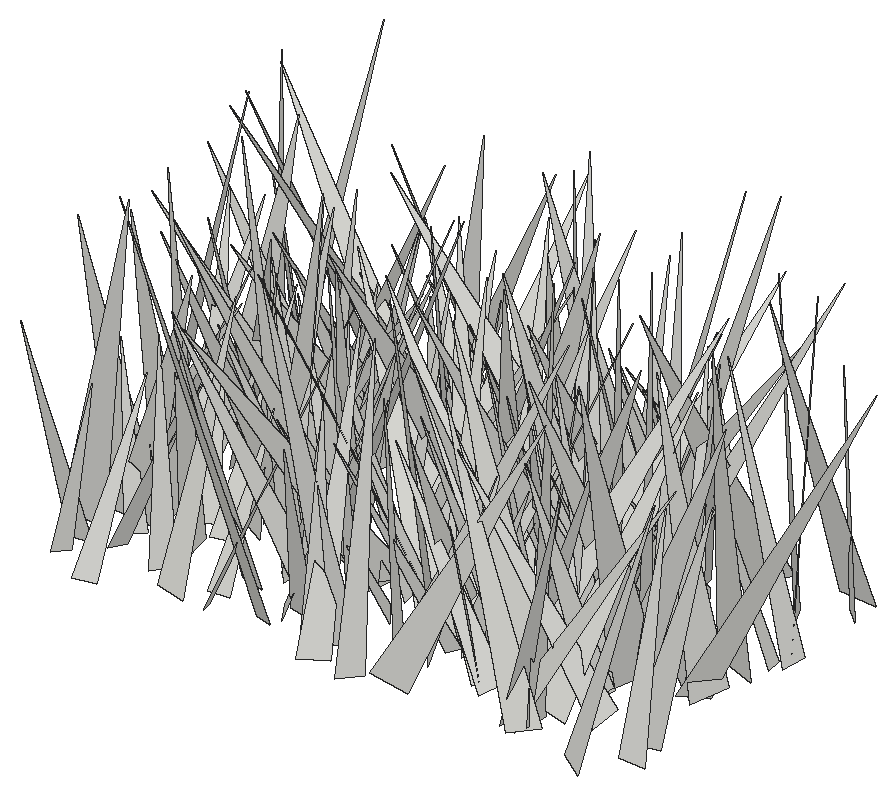
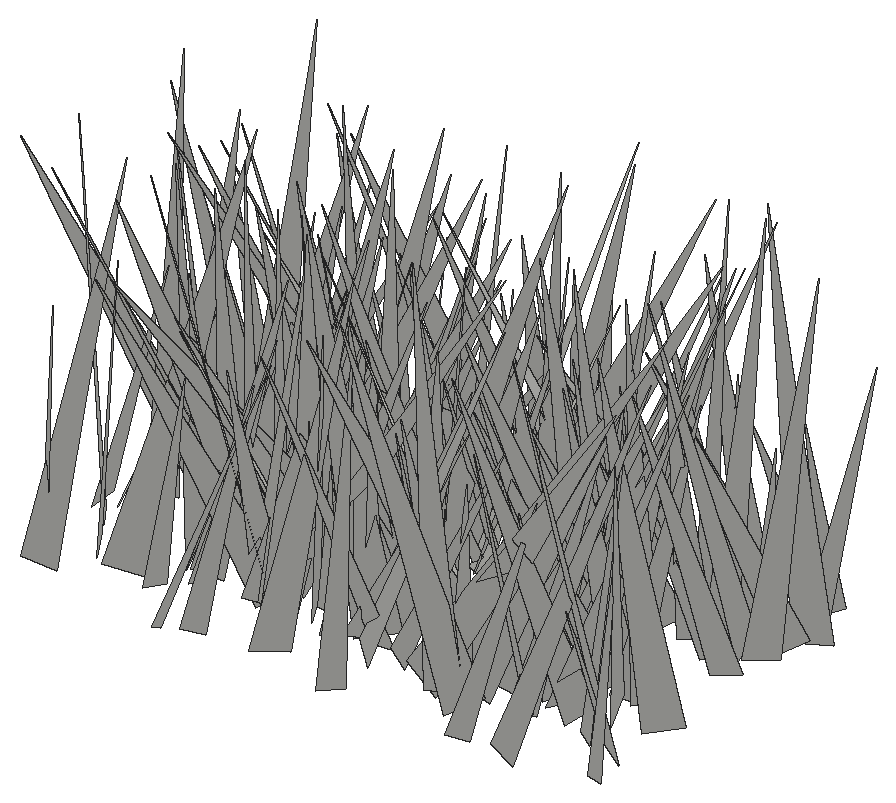
# SketchUp Ruby script. Lengths in inches.
U = 1.inch
M = Sketchup.active_model
def pt(a) = Geom::Point3d.new(a.map { |v| v * U })
def face(e, loops, mat)
  f = e.add_face(loops[0].map { |a| pt(a) })
  loops[1..].each { |l| e.add_face(l.map { |a| pt(a) }).erase! }
  f.material = f.back_material = mat if mat
  f
end
# faces: each face lists its corners as indices into pts; further lists are holes
def faces(e, pts, list, mat = nil) = list.each { |f| face(e, (f[0].is_a?(Array) ? f : [f]).map { |l| l.map { |i| pts[i] } }, mat) }
# xy, xz, yz: faces in a plane at the given z, y or x. An outline is a flat list of corners, or four numbers for a rectangle; further outlines are holes
def ring(l) = l.size == 4 ? [[l[0], l[1]], [l[2], l[1]], [l[2], l[3]], [l[0], l[3]]] : l.each_slice(2).to_a
def flat(e, list, mat, &to3) = list.each { |f| face(e, (f[0].is_a?(Array) ? f : [f]).map { |l| ring(l).map { |u, v| to3.(u, v) } }, mat) }
def xy(e, z, list, mat = nil) = flat(e, list, mat) { |x, y| [x, y, z] }
def xz(e, y, list, mat = nil) = flat(e, list, mat) { |x, z| [x, y, z] }
def yz(e, x, list, mat = nil) = flat(e, list, mat) { |y, z| [x, y, z] }
def lines(e, pts, list) = list.each { |a, b| e.add_line(pt(pts[a]), pt(pts[b])) }
# prism: a flat outline (further loops are holes) pulled along v
def prism(e, loops, v, mat = nil)
  f = face(e, loops, mat); d = Geom::Vector3d.new(v.map { |x| x * U })
  f.pushpull(f.normal.samedirection?(d) ? d.length : -d.length)
end
def box(e, o, s, mat = nil) = prism(e, [[o, [o[0] + s[0], o[1], o[2]], [o[0] + s[0], o[1] + s[1], o[2]], [o[0], o[1] + s[1], o[2]]]], [0, 0, s[2]], mat)
def at(x, y, z, deg = 0) = Geom::Transformation.translation(pt([x, y, z])) * Geom::Transformation.rotation(ORIGIN, Z_AXIS, deg.degrees)
def axes(o, x, y, z) = Geom::Transformation.new([*x, 0, *y, 0, *z, 0, *pt(o).to_a, 1])
def part(name) = M.definitions.add(name)
# library, detail: a bought-in or finely detailed component or shape, given as its bounding box
def library(name, o, s) = part(name).tap { |d| box(d.entities, o, s) }
def detail(e, o, s) = box(e.add_group.entities, o, s)
def put(e, d, t, mat = nil) = e.add_instance(d, t).tap { |i| i.material = mat if mat }
def group(e, t, mat = nil) = e.add_group.tap { |g| g.transformation = t; g.material = mat if mat }.entities
root = M.entities
c1 = part("fur_instance\#9")
p = [[0.8125,0,1.79],[0.67,-0.02,1.48],[0,-0.11,0],[0,0.11,0]]
faces(c1.entities,p,[[0,1,2,3]])
put(root,c1,axes([545.91,126.66,-21.86],[5.53978,-0.90724,0.62547],[-0.85463,-5.56113,-0.49688],[-0.69563,-0.39269,5.59154]))
put(root,c1,axes([535.66,127.86,-21.86],[0.2783,-5.0487,0.14304],[-4.93686,-0.24166,1.07529],[1.0664,0.19877,4.94071]))
put(root,c1,axes([526.28,127.23,-21.86],[-0.19346,-4.85951,0.89963],[-4.92735,0.1202,-0.41034],[-0.38132,0.91231,4.84602]))
put(root,c1,axes([549.55,125.37,-21.86],[2.91311,4.64162,1.0633],[4.76072,-2.81168,-0.76908],[0.10392,-1.30816,5.4258]))
put(root,c1,axes([526.26,126.17,-21.86],[3.08181,-1.73974,0.98019],[-1.88437,-3.1302,0.36886],[-0.66077,0.81254,3.51969]))
put(root,c1,axes([546.97,125.95,-21.66],[-2.40654,5.51072,1.54274],[5.60544,1.9331,1.83892],[-1.15197,-2.10585,5.72519]))
put(root,c1,axes([528.22,124.99,-21.86],[-2.24412,3.20659,0.81725],[3.00578,2.38826,-1.11699],[1.38398,0.01256,3.75108]))
put(root,c1,axes([538.11,126.98,-21.86],[-0.62718,-6.98929,2.39617],[-7.29856,0.2117,-1.29283],[-1.15016,2.46782,6.89725]))
put(root,c1,axes([540.98,125.93,-21.86],[3.61026,-5.57217,1.81458],[-5.57053,-2.60139,3.09478],[1.81959,3.09184,5.87413]))
put(root,c1,axes([537.15,126.65,-21.86],[-2.61332,3.50076,2.27341],[3.90248,3.00092,-0.13507],[1.48133,-1.72983,4.36652]))
put(root,c1,axes([534.79,126.73,-21.86],[-5.1387,-6.17044,1.38685],[-6.22365,4.61615,-2.52214],[-1.12419,2.64967,7.62361]))
put(root,c1,axes([542.95,128.45,-21.86],[-2.708,-3.38854,1.07596],[-2.8715,2.88211,1.84961],[2.09627,-0.42942,3.92357]))
put(root,c1,axes([539.9,125.13,-21.66],[-5.67085,1.89535,1.35099],[1.57668,5.74544,-1.44226],[1.71219,0.98676,5.80265]))
put(root,c1,axes([532.86,128.52,-21.86],[-1.81224,-5.34948,0.90018],[-5.42401,1.80193,-0.21131],[0.08596,0.92064,5.64415]))
put(root,c1,axes([525.4,128.48,-21.86],[1.45469,-7.67033,1.86376],[-7.74266,-1.0178,1.85445],[1.53584,2.13396,7.5836]))
put(root,c1,axes([531.04,126.22,-21.86],[0.94432,5.62245,1.27282],[5.76049,-0.87093,-0.42662],[0.22085,-1.32412,5.68522]))
put(root,c1,axes([548.68,128.33,-21.66],[-5.67147,0.82087,0.04901],[0.80443,5.46726,1.5178],[-0.17066,-1.50898,5.5259]))
put(root,c1,axes([545.83,126.66,-21.86],[3.84668,4.92623,0.09388],[4.62666,-3.57049,-2.21792],[1.69428,-1.43435,5.84342]))
put(root,c1,axes([551.09,126.8,-21.86],[-0.27729,4.76979,1.49646],[4.98187,0.38774,-0.31274],[0.41383,-1.47171,4.7676]))
put(root,c1,axes([534.89,129.3125,-21.86],[-6.28485,-0.79991,0.77187],[-0.56549,6.11624,1.73401],[0.95701,-1.63912,6.09364]))
put(root,c1,axes([536.53,131.54,-21.86],[4.16443,-6.48584,0.7003],[-5.50995,-3.94185,-3.74183],[-3.49241,-1.51483,6.7385]))
put(root,c1,axes([529.8,127.38,-21.86],[3.42061,-2.16163,2.16053],[-2.46149,-3.8706,0.02453],[-1.81151,1.17767,4.04631]))
put(root,c1,axes([544.05,127.85,-21.86],[-4.37284,2.10544,0.41102],[2.13916,4.20984,1.19366],[-0.16073,-1.25217,4.70423]))
put(root,c1,axes([541.25,130.33,-21.66],[5.27025,-2.47106,0.85487],[-2.00329,-5.05203,-2.25305],[-1.68041,-1.72721,5.36707]))
put(root,c1,axes([537.88,125.61,-21.86],[-5.09281,3.29268,0.78292],[3.01884,5.05892,-1.63872],[1.53013,0.9783,5.83893]))
put(root,c1,axes([537.95,129.79,-21.86],[-3.80651,-3.12707,0.03174],[-3.06593,3.74155,0.93273],[0.61617,-0.70095,4.83716]))
put(root,c1,axes([540.84,128.29,-21.86],[3.81482,2.67004,0.71919],[2.75746,-3.58156,-1.32965],[0.20681,-1.49748,4.4625]))
put(root,c1,axes([532.44,127.17,-21.86],[-1.29453,3.3269,0.92168],[3.25121,1.50588,-0.8692],[1.16077,-0.50757,3.46245]))
put(root,c1,axes([550.69,127.96,-21.86],[3.34726,-4.07819,1.53745],[-4.35777,-3.09938,1.26621],[0.07255,1.99042,5.12177]))
put(root,c1,axes([547.47,129.55,-21.66],[-4.78026,1.17069,2.19317],[1.89155,4.79719,1.56216],[1.61324,-2.15588,4.66702]))
put(root,c1,axes([526.73,129.53,-21.86],[2.49015,-6.48815,0.76577],[-6.33726,-2.19962,1.97082],[1.58797,1.39602,6.66429]))
put(root,c1,axes([545.3,128.73,-21.66],[3.76435,-5.16952,3.38659],[-5.24976,-4.76711,-1.44149],[-3.26082,1.70703,6.23028]))
put(root,c1,axes([540.42,127.59,-21.86],[4.07945,6.65627,1.20942],[6.56454,-3.55321,-2.58689],[1.63565,-2.3408,7.36585]))
put(root,c1,axes([539.65,128.14,-21.86],[-4.30965,-1.39305,1.63599],[-1.58025,4.5392,-0.29767],[1.45598,0.80324,4.51941]))
put(root,c1,axes([527.98,130.34,-21.66],[6.98441,-2.34407,2.00985],[-1.86712,-7.16517,-1.86827],[-2.45928,-1.21733,7.12645]))
put(root,c1,axes([529.87,128.97,-21.86],[-7.27615,-1.41209,3.18772],[-1.2687,7.94356,0.62294],[3.24745,-0.06052,7.38568]))
put(root,c1,axes([541.52,128.89,-21.66],[-1.12844,-4.06047,0.83548],[-3.60524,0.5338,-2.27512],[-2.04639,1.29864,3.54749]))
put(root,c1,axes([547.48,131.46,-21.86],[6.81384,-4.6319,0.82302],[-4.34734,-6.75311,-2.01405],[-1.7979,-1.22528,7.98915]))
put(root,c1,axes([546.91,126.72,-21.66],[-7.37531,-1.40171,2.74866],[-2.16749,7.42249,-2.03071],[2.19589,2.61858,7.22747]))
put(root,c1,axes([543.5,128.16,-21.86],[-3.62089,2.64212,0.01483],[2.58278,3.53416,0.96476],[-0.55698,-0.78788,4.37731]))
put(root,c1,axes([537.35,132.18,-21.66],[-4.65731,-6.85842,0.0184],[-6.74044,4.58127,1.51895],[1.26677,-0.83835,8.14992]))
put(root,c1,axes([525.89,130.72,-21.66],[5.91516,-3.3432,1.65321],[-2.9566,-6.09276,-1.74243],[-2.27346,-0.77492,6.56735]))
put(root,c1,axes([543.75,129.52,-21.86],[-0.61117,-4.98438,1.28841],[-4.9544,0.21679,-1.51148],[-1.3993,1.40945,4.78884]))
put(root,c1,axes([539.55,130.21,-21.86],[-4.05006,-5.82532,2.03849],[-5.82326,4.4146,1.04584],[2.04438,1.03428,7.01738]))
put(root,c1,axes([527.52,128.74,-21.86],[-2.21806,2.84038,1.31516],[3.07662,2.27502,0.2754],[0.57601,-1.21396,3.59328]))
put(root,c1,axes([537.99,127.83,-21.66],[-6.10428,-1.79449,1.71008],[-2.20054,6.01533,-1.54278],[1.14113,2.0006,6.1727]))
put(root,c1,axes([527.43,127.86,-21.86],[4.11341,0.99659,0.14821],[0.94897,-4.04143,0.83763],[-0.33855,0.78037,4.1487]))
put(root,c1,axes([541.73,129.39,-21.66],[0.78956,-4.05986,1.16414],[-3.93825,-0.27989,1.69498],[1.52574,1.37851,3.77266]))
put(root,c1,axes([544.34,129.38,-21.86],[5.3173,-1.56529,0.48292],[-1.59322,-5.32309,0.28875],[-0.38078,0.41424,5.53538]))
put(root,c1,axes([527.8,127.38,-21.66],[5.78446,0.51407,0.77192],[0.25637,-5.57234,1.78981],[-0.89129,1.73346,5.52457]))
put(root,c1,axes([532.67,126.25,-21.86],[5.39727,3.08007,0.18691],[2.81936,-5.07536,2.22356],[-1.25418,1.84558,5.80286]))
put(root,c1,axes([546.83,127.5,-21.66],[0.07577,6.70614,0.84141],[6.48392,0.16538,-1.90197],[1.90764,-0.82847,6.43122]))
put(root,c1,axes([541.76,130.47,-21.86],[0.99148,-3.49866,0.36174],[-3.47594,-0.91715,0.65665],[0.53788,0.52224,3.57665]))
put(root,c1,axes([535.07,131.43,-21.86],[-0.95701,-7.3765,1.52863],[-7.35851,1.24531,1.40248],[1.61303,1.30453,7.30491]))
put(root,c1,axes([525.54,129.35,-21.66],[4.06898,-3.86093,0.67624],[-3.71406,-3.48612,2.44405],[1.25293,2.20473,5.04877]))
put(root,c1,axes([536.17,131.25,-21.86],[-0.88156,-7.55851,1.51866],[-6.98391,0.13553,-3.37952],[-3.26533,1.75074,6.81814]))
put(root,c1,axes([545.95,128.66,-21.86],[-5.8174,-1.77979,0.63377],[-1.88895,5.44209,-2.05595],[-0.03436,2.15114,5.72563]))
put(root,c1,axes([546.76,133.03,-21.86],[4.80853,-5.64104,1.01196],[-5.19564,-4.8483,-2.3381],[-2.41883,-0.80002,7.03396]))
put(root,c1,axes([535.25,127.27,-21.66],[6.47525,4.61232,0.40047],[4.47579,-6.41261,1.48613],[-1.18373,0.98374,7.80985]))
put(root,c1,axes([531.86,132.4,-21.86],[0.11863,-7.1905,0.64579],[-7.08435,-0.24031,-1.37429],[-1.39009,0.61104,7.05894]))
put(root,c1,axes([547.37,129.81,-21.86],[-5.94659,0.26274,1.16381],[0.1992,6.05181,-0.34844],[1.17635,0.30341,5.94219]))
put(root,c1,axes([541.85,132.21,-21.86],[-5.8383,-2.13052,1.19785],[-1.77007,5.82456,1.73238],[1.68547,-1.263,5.96857]))
put(root,c1,axes([542.11,129.29,-21.86],[-2.40389,3.30252,0.08348],[3.28439,2.37806,0.4999],[-0.35549,-0.36124,4.05406]))
put(root,c1,axes([547.38,131.37,-21.66],[1.03631,-6.95808,1.71035],[-6.57848,-0.23906,3.0134],[2.83968,1.98547,6.35675]))
put(root,c1,axes([545.26,130.74,-21.86],[3.00481,-2.76961,0.12717],[-2.71494,-2.90128,0.96303],[0.56213,0.79222,3.97142]))
put(root,c1,axes([539.18,130.71,-21.86],[-0.30638,-3.92044,1.36874],[-3.76361,-0.31774,-1.75256],[-1.75458,1.36615,3.52026]))
put(root,c1,axes([544.57,129.3,-21.86],[3.86177,3.77021,1.4507],[3.73701,-4.09632,0.69796],[-1.5342,-0.48777,5.35169]))
put(root,c1,axes([543.65,130.46,-21.86],[-6.06762,4.08752,0.30456],[4.00596,5.79855,1.98636],[-0.86766,-1.81261,7.04117]))
put(root,c1,axes([533.8125,131.25,-21.66],[-0.35504,-4.51922,1.36303],[-4.31721,-0.2418,-1.92625],[-1.90863,1.3876,4.10353]))
put(root,c1,axes([537.69,131.45,-21.86],[-5.30182,-0.75056,0.88287],[-0.65483,5.35184,0.61739],[0.95603,-0.49663,5.31898]))
put(root,c1,axes([533.7,129.9,-21.86],[-7.85501,-1.13743,1.66782],[-1.3997,7.89692,-1.20666],[1.45472,1.45652,7.84468]))
put(root,c1,axes([544.45,128.0625,-21.86],[1.49345,8.09623,0.02611],[7.76227,-1.42429,-2.34489],[2.30146,-0.44999,7.89182]))
put(root,c1,axes([535.08,129.1,-21.86],[7.43701,2.08557,1.03262],[1.85087,-7.39668,1.60887],[-1.41074,1.29018,7.55449]))
put(root,c1,axes([534.76,129.44,-21.86],[-6.83852,1.49302,2.47832],[0.97247,7.17644,-1.63995],[2.72497,1.18576,6.80477]))
put(root,c1,axes([550.23,132.17,-21.86],[-6.01027,1.97565,2.91231],[2.62602,6.35479,1.10849],[2.3428,-2.05464,6.22879]))
put(root,c1,axes([534.01,132.39,-21.86],[3.60736,-4.41491,0.21347],[-4.38405,-3.53869,0.89879],[0.56311,0.73233,5.62998]))
put(root,c1,axes([543.74,133.88,-21.86],[1.64942,-7.33453,1.1804],[-6.83961,-1.97125,-2.69132],[-2.89974,0.47759,7.01946]))
put(root,c1,axes([533.58,129.57,-21.66],[3.9731,1.20771,1.01378],[0.70264,-3.81635,1.79266],[-1.41159,1.49959,3.74573]))
put(root,c1,axes([540.6,130.62,-21.86],[0.79551,4.29487,0.6755],[4.10301,-0.51451,-1.56067],[1.4379,-0.90797,4.07959]))
put(root,c1,axes([545.96,133.21,-21.86],[-3.41692,-2.65793,0.41527],[-2.50813,3.39027,1.06197],[0.9728,-0.5949,4.19669]))
put(root,c1,axes([541.99,133.5625,-21.66],[-0.85203,-5.57664,0.61964],[-5.3803,0.98986,1.51043],[1.59225,0.36067,5.43539]))
put(root,c1,axes([527.5625,131.52,-21.86],[0.91676,-3.52562,1.5814],[-3.59518,-0.18259,1.67709],[1.41617,1.81877,3.23385]))
put(root,c1,axes([540.4,129.98,-21.86],[-0.0106,6.43156,0.96228],[6.47441,-0.07994,0.60561],[-0.61077,-0.95901,6.403]))
put(root,c1,axes([530.67,131.32,-21.86],[-2.24155,-3.80564,2.54295],[-4.42537,2.52493,-0.12217],[1.16862,2.26183,4.41503]))
put(root,c1,axes([542.01,129.26,-21.66],[5.76242,3.50846,0.12226],[3.39302,-5.62636,1.53663],[-0.90093,1.2508,6.56914]))
put(root,c1,axes([539.1875,130.89,-21.86],[-3.95209,5.35159,0.47213],[5.26841,3.74586,1.6413],[-1.05182,-1.34553,6.44707]))
put(root,c1,axes([528.77,130.73,-21.86],[-2.92394,5.35838,1.35906],[5.44647,3.05552,-0.32925],[0.94614,-1.02969,6.09534]))
put(root,c1,axes([531.34,135.57,-21.86],[-7.53778,-2.79862,0.78068],[-2.32716,7.11502,3.03655],[1.73954,-2.60846,7.44512]))
put(root,c1,axes([549.75,134.18,-21.86],[-1.05079,-7.8114,1.55453],[-7.7743,1.34665,1.51176],[1.73053,1.30661,7.73542]))
put(root,c1,axes([530.13,133.37,-21.86],[-2.71876,-5.31687,1.33657],[-5.469,2.73415,-0.24823],[0.3815,1.3048,5.9665]))
put(root,c1,axes([526.8125,130.41,-21.66],[7.21368,2.51232,2.17903],[2.05011,-7.45745,1.81123],[-2.61859,1.08246,7.42081]))
put(root,c1,axes([530.16,130.3,-21.86],[-3.50119,3.09472,0.56001],[2.74674,3.41714,-1.71109],[1.53177,0.94611,4.34831]))
put(root,c1,axes([537.53,131.625,-21.86],[0.85166,3.52496,0.51911],[3.494,-0.72175,-0.83136],[0.69768,-0.68839,3.5298]))
put(root,c1,axes([543.71,134.28,-21.86],[3.93699,-6.31061,2.13001],[-6.14082,-4.39732,-1.67764],[-2.57895,0.83692,7.24632]))
put(root,c1,axes([537.04,136.71,-21.66],[4.97759,-6.71856,0.2944],[-6.18791,-4.7191,-3.07278],[-2.63353,-1.61035,7.77647]))
put(root,c1,axes([548.67,132.4375,-21.86],[-3.30417,-4.76212,3.2823],[-5.25525,4.05058,0.5865],[2.41528,2.29867,5.7664]))
put(root,c1,axes([530.75,132.79,-21.86],[6.63487,-1.65212,1.91106],[-1.73662,-6.8834,0.0785],[-1.83462,0.54083,6.83702]))
put(root,c1,axes([531.94,132.67,-21.86],[-4.97089,0.8761,1.32855],[0.91857,5.13772,0.0489],[1.29955,-0.28038,5.04727]))
put(root,c1,axes([540.04,131.45,-21.86],[4.12915,-1.39251,2.24683],[-2.1688,-4.1671,1.40312],[-1.51116,2.17563,4.12556]))
put(root,c1,axes([543.69,133.71,-21.86],[-5.54142,2.04017,2.02802],[2.50487,5.58649,1.22443],[1.41448,-1.90035,5.77671]))
put(root,c1,axes([531.92,131.91,-21.86],[-3.26703,2.9675,0.38966],[2.97957,3.27925,0.00816],[0.28293,-0.26806,4.41355]))
put(root,c1,axes([539.02,135.18,-21.66],[7.15666,-2.1147,0.99823],[-1.83229,-7.06792,-1.83669],[-1.45298,-1.50292,7.233]))
put(root,c1,axes([527.1875,135.36,-21.86],[6.92696,-1.79403,0.01467],[-1.72828,-6.68834,-1.86567],[-0.48147,-1.80253,6.90801]))
put(root,c1,axes([547.54,131.93,-21.86],[-6.71268,-1.89599,2.76742],[-2.51748,6.93875,-1.3526],[2.21714,2.13833,6.8429]))
put(root,c1,axes([540.52,135.47,-21.66],[-1.15105,-5.30671,0.17],[-5.09537,1.15297,1.49093],[1.49242,-0.15644,5.22142]))
put(root,c1,axes([531.79,131.72,-21.86],[0.8824,6.11345,1.2337],[6.18895,-1.01221,0.58924],[-0.77016,-1.12963,6.14863]))
put(root,c1,axes([538.15,132.59,-21.86],[7.40622,-0.19557,0.80001],[-0.28757,-7.3972,0.85392],[-0.77173,0.87956,7.35943]))
put(root,c1,axes([532.19,132.56,-21.66],[5.41003,-2.25588,0.78895],[-2.38957,-5.13634,1.69936],[-0.03699,1.87321,5.60977]))
put(root,c1,axes([526.18,132.3125,-21.66],[-0.72846,5.64896,1.65026],[5.62241,1.15927,-1.48642],[1.73859,-1.38206,5.49837]))
put(root,c1,axes([549.83,131.79,-21.86],[6.83257,-2.01041,0.78824],[-2.1593,-6.33413,2.56189],[0.022,2.68032,6.64549]))
put(root,c1,axes([528.02,135.61,-21.86],[1.38462,-5.25865,0.1546],[-5.22749,-1.39323,-0.57157],[-0.5921,0.00308,5.40776]))
put(root,c1,axes([537.02,131.32,-21.66],[1.91748,5.33638,0.31642],[5.10909,-1.9283,1.55969],[-1.57297,0.24194,5.4517]))
put(root,c1,axes([541.4375,134.98,-21.86],[3.81645,-5.44593,0.15233],[-5.28758,-3.65777,1.70554],[1.31259,1.09964,6.42764]))
put(root,c1,axes([537.46,134.09,-21.86],[-5.46396,-3.21591,2.3792],[-3.43589,5.83542,-0.00311],[2.04873,1.20967,6.3401]))
put(root,c1,axes([541.67,135.38,-21.86],[-1.836,-5.36618,0.72675],[-5.38286,1.72484,-0.86298],[-0.59066,0.96126,5.60554]))
put(root,c1,axes([544.51,134.14,-21.86],[5.88559,1.89129,2.87248],[1.95642,-6.52369,0.2867],[-2.82853,-0.57687,6.17535]))
put(root,c1,axes([532.28,133.96,-21.86],[-3.96056,0.86775,0.15545],[0.85071,3.94968,-0.37345],[0.23119,0.33194,4.03727]))
put(root,c1,axes([533.17,133.45,-21.86],[-3.9297,0.38452,0.60241],[0.18265,3.7953,-1.23109],[0.69093,1.18368,3.75164]))
put(root,c1,axes([535.19,134.89,-21.66],[5.77692,4.11347,0.10405],[3.90568,-5.42514,-2.37018],[1.29504,-1.98782,6.68399]))
put(root,c1,axes([529.42,134.15,-21.86],[4.47757,-3.00826,2.16701],[-3.51648,-4.52249,0.98776],[-1.1747,2.07164,5.30307]))
put(root,c1,axes([545.58,137.26,-21.66],[6.93671,-0.62868,0.23505],[-0.51232,-6.5363,-2.3628],[-0.4336,-2.33453,6.55213]))
put(root,c1,axes([547.41,133.11,-21.66],[1.24745,7.40868,1.63783],[7.39275,-1.56046,1.42803],[-1.70827,-1.34297,7.376]))
put(root,c1,axes([545.1,133,-21.86],[4.06306,2.1594,0.43468],[1.91332,-3.91175,1.54848],[-1.0914,1.18135,4.33286]))
put(root,c1,axes([548.25,133.47,-21.86],[-0.40963,5.6712,0.85204],[5.69515,0.30195,0.72827],[-0.67361,-0.89587,5.63914]))
put(root,c1,axes([545.93,137.53,-21.86],[-3.33896,-2.6162,0.26799],[-2.1089,2.92233,2.25332],[1.57125,-1.6372,3.59384]))
put(root,c1,axes([532.65,133.34,-21.66],[5.29795,0.17393,1.896],[-0.4687,-5.31448,1.7972],[-1.84537,1.84915,4.98684]))
put(root,c1,axes([531.67,137.9,-21.66],[2.44843,-5.51273,0.60157],[-4.8536,-2.44839,-2.68234],[-2.6823,-0.60174,5.40279]))
put(root,c1,axes([541.93,138.4,-21.66],[4.15216,-5.25606,0.30062],[-4.95254,-4.0295,-2.04756],[-1.78575,-1.04593,6.37763]))
put(root,c1,axes([539.2,134.86,-21.66],[-0.86303,4.80618,1.97762],[4.83833,1.47497,-1.47315],[1.8976,-1.57489,4.65553]))
put(root,c1,axes([529,135.29,-21.86],[4.24231,-3.44067,0.07958],[-3.18347,-3.87509,2.16585],[1.3077,1.72835,5.01442]))
put(root,c1,axes([537.81,134.17,-21.86],[-5.07407,3.61415,0.85454],[3.5922,5.14344,-0.42375],[0.94256,-0.14624,6.2152]))
put(root,c1,axes([550.65,135.23,-21.86],[-4.94313,-1.68267,0.02369],[-1.64372,4.81198,-1.18726],[-0.36076,1.13137,5.08492]))
put(root,c1,axes([541.55,135.9,-21.86],[5.6621,3.46946,2.68851],[3.90579,-5.98471,-0.5026],[-2.00251,-1.86297,6.62147]))
put(root,c1,axes([546.99,139.58,-21.66],[4.52461,-6.7861,0.00105],[-6.53347,-4.35651,-2.20405],[-1.83437,-1.22185,7.85273]))
put(root,c1,axes([539.01,134.35,-21.66],[-2.13966,5.92839,0.3544],[5.56639,1.87053,2.31645],[-2.07043,-1.09766,5.86157]))
put(root,c1,axes([540.25,133.81,-21.86],[-1.0825,6.58238,0.66021],[6.6005,1.02978,0.55528],[-0.44383,-0.73975,6.64764]))
put(root,c1,axes([542.28,138.35,-21.66],[-3.66849,-5.82093,1.22872],[-5.44278,3.86666,2.06783],[2.40191,-0.1285,6.56241]))
put(root,c1,axes([537.57,137.4,-21.86],[3.43501,-7.39782,1.03394],[-7.28345,-3.06455,2.27067],[1.65774,1.86463,7.83397]))
put(root,c1,axes([540.92,138.71,-21.86],[3.46816,-3.92613,0.03464],[-3.68547,-3.27126,-1.77763],[-1.35388,-1.15247,4.92774]))
put(root,c1,axes([541.65,137.58,-21.66],[-7.78216,2.50032,0.23977],[2.4235,7.26917,2.85602],[-0.66011,-2.78901,7.65877]))
put(root,c1,axes([551.06,135.8125,-21.86],[-5.68888,-0.08485,0.69236],[-0.12916,5.71868,-0.36046],[0.68548,0.37338,5.67808]))
put(root,c1,axes([544.89,137.76,-21.86],[1.51534,-5.37644,0.92666],[-5.31705,-1.67082,-0.99923],[-1.22223,0.60275,5.49581]))
put(root,c1,axes([529.37,137.58,-21.66],[-6.5147,0.26004,1.16019],[0.55336,6.38259,1.67669],[1.05235,-1.74639,6.3006]))
put(root,c1,axes([542.7,134.1,-21.86],[5.57667,1.59527,0.3002],[1.43066,-5.3377,1.78788],[-0.76695,1.64269,5.51794]))
put(root,c1,axes([532.35,138.51,-21.86],[-0.06223,-5.95217,0.13196],[-5.73579,0.02457,-1.59678],[-1.59576,0.14382,5.73432]))
put(root,c1,axes([550.26,136.71,-21.86],[-5.21121,-4.35385,3.58957],[-4.50193,6.15376,0.92827],[3.40202,1.4741,6.72689]))
put(root,c1,axes([543.8,133.88,-21.86],[4.07971,3.91858,0.07723],[3.79656,-3.97882,1.32677],[-0.97331,0.90496,5.499]))
put(root,c1,axes([542.94,134.38,-21.86],[-0.59735,8.07244,1.41711],[8.08686,0.34954,1.4177],[-1.33238,-1.49761,7.96939]))
put(root,c1,axes([525.61,136.5,-21.86],[4.4224,-5.22883,1.99199],[-5.58659,-4.26873,1.19762],[-0.31423,2.30295,6.7427]))
put(root,c1,axes([543.53,132.53,-21.86],[-3.48939,6.7058,0.49493],[5.71017,3.24965,-3.77124],[3.55058,1.36403,6.55144]))
put(root,c1,axes([538.36,136.56,-21.86],[-3.33469,1.40616,1.82105],[1.56398,3.73727,-0.02186],[1.68745,-0.685,3.61897]))
put(root,c1,axes([530.26,138.54,-21.86],[2.83348,-4.00549,0.52306],[-3.76222,-2.8494,-1.43972],[-1.47079,-0.42795,4.69039]))
put(root,c1,axes([544.79,135.1,-21.86],[4.68977,6.59581,0.10077],[6.41242,-4.52929,-1.96857],[1.54784,-1.22048,7.85006]))
put(root,c1,axes([534.22,139.1875,-21.66],[-2.23996,-8.03771,0.28468],[-7.44594,1.96073,-3.22749],[-3.04036,1.11981,7.69451]))
put(root,c1,axes([538.84,138.47,-21.86],[3.04717,-2.22298,0.43436],[-2.028,-3.00193,-1.13631],[-1.00873,-0.67996,3.59662]))
put(root,c1,axes([544.81,138.3125,-21.86],[-4.67386,-0.0885,1.27111],[0.2568,4.66814,1.26925],[1.24804,-1.29194,4.49909]))
put(root,c1,axes([535.48,136.86,-21.86],[4.00682,1.30969,1.18737],[1.29487,-4.17692,0.23764],[-1.20352,-0.13365,4.20874]))
put(root,c1,axes([538.14,137.95,-21.86],[-4.58905,2.11277,0.48874],[2.15665,4.32669,1.54618],[-0.22698,-1.60562,4.80963]))
put(root,c1,axes([545.27,134.55,-21.66],[7.73551,0.03019,2.73159],[-1.01366,-7.58581,2.95441],[-2.53672,3.12332,7.14916]))
put(root,c1,axes([530.04,137.06,-21.86],[3.18405,-1.52738,1.26596],[-1.78098,-3.25535,0.55182],[-0.87386,1.06936,3.48806]))
put(root,c1,axes([535.05,136.71,-21.86],[-1.4542,4.67664,1.33998],[4.76533,1.65076,-0.58976],[0.97884,-1.08869,4.86188]))
put(root,c1,axes([527.4,138.64,-21.86],[-3.25628,-4.53556,1.56998],[-4.60157,3.48952,0.53691],[1.36443,0.94415,5.55755]))
put(root,c1,axes([545.9,137.42,-21.86],[-3.57996,-1.2077,0.30439],[-1.24532,3.48547,-0.8173],[0.0195,0.87192,3.68872]))
put(root,c1,axes([543.23,136.63,-21.86],[5.81873,5.70667,1.51485],[5.84557,-5.86726,-0.35074],[-0.83073,-1.31442,8.14252]))
put(root,c1,axes([537.17,138.7,-21.86],[-5.01465,-5.39389,0.78065],[-5.43536,4.87162,-1.25473],[-0.40033,1.42249,7.25716]))
put(root,c1,axes([535.75,134.96,-21.86],[-2.62249,6.7547,0.84995],[6.3246,2.75431,-2.37468],[2.5195,0.11678,6.84575]))
put(root,c1,axes([539.99,137.19,-21.86],[-0.46969,3.55211,0.73396],[3.59032,0.35011,0.60316],[-0.51554,-0.79795,3.53189]))
put(root,c1,axes([533.2,138.29,-21.86],[1.90593,-3.10212,1.28599],[-3.27722,-2.04084,-0.06594],[-0.73267,1.05893,3.64024]))
put(root,c1,axes([535.77,138.56,-21.66],[-2.3451,-4.39084,0.71964],[-4.31416,2.04482,-1.58228],[-1.08875,1.35503,4.71968]))
put(root,c1,axes([534.6,137.08,-21.66],[-4.02573,7.19257,0.41274],[6.48293,3.4104,3.80141],[-3.14246,-2.17854,7.31361]))
put(root,c1,axes([528.5,137.48,-21.86],[6.61677,-1.08212,0.53072],[-1.15649,-6.53431,1.0953],[-0.3394,1.16883,6.6146]))
put(root,c1,axes([541.81,137.9,-21.66],[4.55,-4.60588,0.41001],[-4.16176,-3.82822,3.1795],[2.01545,2.49305,5.6398]))
put(root,c1,axes([533.07,139.41,-21.66],[0.67729,-7.55263,2.0847],[-7.70125,-0.25666,1.57216],[1.44182,2.17688,7.41817]))
put(root,c1,axes([549.94,140.77,-21.86],[-0.40558,-7.48594,0.6627],[-7.51279,0.42075,0.15485],[0.19107,0.65318,7.49532]))
put(root,c1,axes([530.23,138.26,-21.86],[2.95558,3.83246,1.3061],[4.0436,-2.87668,-0.7093],[-0.20723,-1.47175,4.78749]))
put(root,c1,axes([540.48,137.22,-21.86],[-6.12572,-2.31991,2.2614],[-2.97153,5.95041,-1.94497],[1.2907,2.68904,6.25488]))
put(root,c1,axes([527.53,136.67,-21.66],[-6.50203,-1.48304,1.94789],[-2.15091,6.10063,-2.53495],[1.1693,2.97539,6.16846]))
put(root,c1,axes([542.96,136.78,-21.86],[-5.40299,1.91129,1.15946],[1.49374,5.34299,-1.84687],[1.66317,1.41036,5.42535]))
put(root,c1,axes([528.92,141.34,-21.86],[-3.06964,-6.81398,0.3454],[-6.81954,3.05272,-0.38339],[-0.20825,0.47214,7.46364]))
put(root,c1,axes([549.11,138.47,-21.86],[-5.34444,-2.84039,2.21318],[-3.30562,5.4408,-0.99979],[1.42788,1.96442,5.96919]))
put(root,c1,axes([536.9,137.96,-21.86],[1.84734,5.85191,0.92453],[5.8229,-1.61485,-1.41361],[1.09242,-1.28828,5.97153]))
put(root,c1,axes([542.55,141.48,-21.66],[3.43107,-2.8474,0.0502],[-2.64084,-3.2106,-1.6126],[-1.06592,-1.21113,4.15686]))
put(root,c1,axes([545.82,139.48,-21.86],[-3.82053,1.38738,1.41647],[1.59253,3.97908,0.39802],[1.18113,-0.87734,4.0451]))
put(root,c1,axes([530.88,141.37,-21.86],[3.08843,-3.08617,0.55459],[-2.71507,-3.02147,-1.69397],[-1.56857,-0.84658,4.0241]))
put(root,c1,axes([543.73,142.04,-21.66],[-4.54437,-2.07997,0.71062],[-1.49312,4.11891,2.50752],[1.61302,-2.04715,4.32318]))
put(root,c1,axes([539.58,140.91,-21.66],[-6.14349,2.42883,3.06477],[3.31416,6.26335,1.67969],[2.07568,-2.81172,6.38908]))
put(root,c1,axes([532.07,139.5,-21.86],[6.60673,-3.01857,0.44503],[-3.04917,-6.49303,1.22551],[0.11127,1.29906,7.15953]))
put(root,c1,axes([525.34,140.7,-21.86],[-1.38247,-3.90181,0.99129],[-3.91317,1.54858,0.63797],[0.94545,0.70412,4.09003]))
put(root,c1,axes([550.55,139.7,-21.86],[-3.07714,-3.38347,1.94932],[-3.73457,3.27489,-0.21099],[1.14047,1.59489,4.5686]))
put(root,c1,axes([526.62,138.41,-21.86],[1.50713,3.43781,0.3216],[3.3001,-1.53741,0.96906],[-1.01552,0.10596,3.62641]))
put(root,c1,axes([536.23,141.7,-21.66],[5.5268,-1.95543,1.04999],[-1.67194,-5.52102,-1.48142],[-1.45972,-1.07995,5.67227]))
put(root,c1,axes([525.95,138.97,-21.86],[-3.45696,-5.56122,4.74392],[-6.59951,4.63089,0.61955],[3.14299,3.60698,6.51874]))
